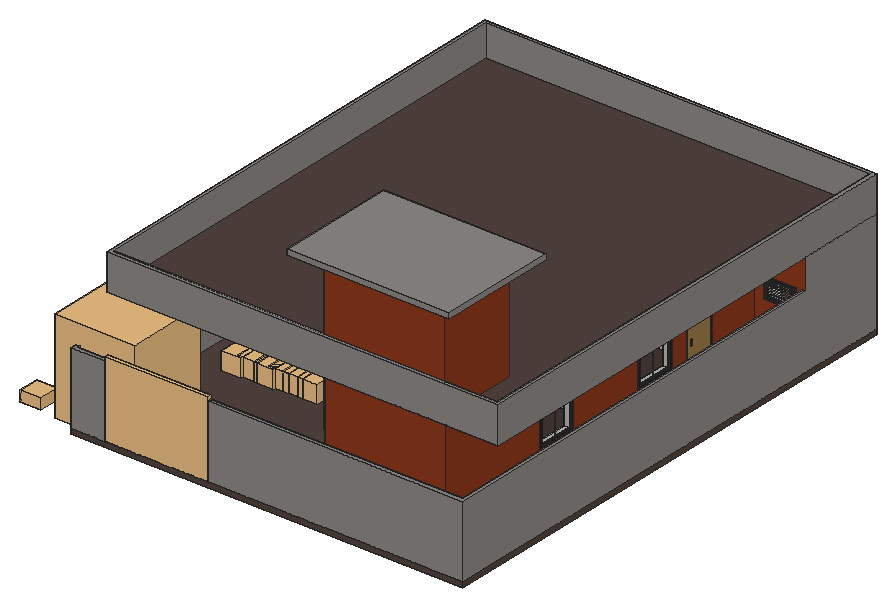
# SketchUp Ruby script. Lengths in inches.
U = 1.inch
M = Sketchup.active_model
def pt(a) = Geom::Point3d.new(a.map { |v| v * U })
def face(e, loops, mat)
  f = e.add_face(loops[0].map { |a| pt(a) })
  loops[1..].each { |l| e.add_face(l.map { |a| pt(a) }).erase! }
  f.material = f.back_material = mat if mat
  f
end
# faces: each face lists its corners as indices into pts; further lists are holes
def faces(e, pts, list, mat = nil) = list.each { |f| face(e, (f[0].is_a?(Array) ? f : [f]).map { |l| l.map { |i| pts[i] } }, mat) }
# xy, xz, yz: faces in a plane at the given z, y or x. An outline is a flat list of corners, or four numbers for a rectangle; further outlines are holes
def ring(l) = l.size == 4 ? [[l[0], l[1]], [l[2], l[1]], [l[2], l[3]], [l[0], l[3]]] : l.each_slice(2).to_a
def flat(e, list, mat, &to3) = list.each { |f| face(e, (f[0].is_a?(Array) ? f : [f]).map { |l| ring(l).map { |u, v| to3.(u, v) } }, mat) }
def xy(e, z, list, mat = nil) = flat(e, list, mat) { |x, y| [x, y, z] }
def xz(e, y, list, mat = nil) = flat(e, list, mat) { |x, z| [x, y, z] }
def yz(e, x, list, mat = nil) = flat(e, list, mat) { |y, z| [x, y, z] }
def lines(e, pts, list) = list.each { |a, b| e.add_line(pt(pts[a]), pt(pts[b])) }
# prism: a flat outline (further loops are holes) pulled along v
def prism(e, loops, v, mat = nil)
  f = face(e, loops, mat); d = Geom::Vector3d.new(v.map { |x| x * U })
  f.pushpull(f.normal.samedirection?(d) ? d.length : -d.length)
end
def box(e, o, s, mat = nil) = prism(e, [[o, [o[0] + s[0], o[1], o[2]], [o[0] + s[0], o[1] + s[1], o[2]], [o[0], o[1] + s[1], o[2]]]], [0, 0, s[2]], mat)
def at(x, y, z, deg = 0) = Geom::Transformation.translation(pt([x, y, z])) * Geom::Transformation.rotation(ORIGIN, Z_AXIS, deg.degrees)
def axes(o, x, y, z) = Geom::Transformation.new([*x, 0, *y, 0, *z, 0, *pt(o).to_a, 1])
def part(name) = M.definitions.add(name)
# library, detail: a bought-in or finely detailed component or shape, given as its bounding box
def library(name, o, s) = part(name).tap { |d| box(d.entities, o, s) }
def detail(e, o, s) = box(e.add_group.entities, o, s)
def put(e, d, t, mat = nil) = e.add_instance(d, t).tap { |i| i.material = mat if mat }
def group(e, t, mat = nil) = e.add_group.tap { |g| g.transformation = t; g.material = mat if mat }.entities
root = M.entities
M.materials.add("Aluminium Black Anodized 15cm").color = [38, 38, 38]
M.materials.add("Glass Yellow 001").color = [0, 0, 0]
M.materials["Glass Yellow 001"].alpha = 0.1
M.materials.add("Marble Emperador Dark 150cm").color = [81, 67, 62]
M.materials.add("Oak Northland Highgloss 300cm").color = [154, 122, 73]
M.materials.add("Wall Paint Autumn Maple Semigloss 300cm").color = [140, 56, 28]
M.materials.add("Wall Paint Poised Taupe Semigloss 300cm").color = [140, 135, 132]
c1 = library("Schefflera arboricola 003",[-47.85,-46.83,-0.79],[92.88,94.95,107.86])
c2 = library("Scabiosa atropurpurea 005",[-19.05,-18.08,-0.55],[34.7,36.31,33.14])
c3 = library("Skimmia japonica Rubella 004",[-17.08,-16.64,-0.26],[33.2,34.59,28.81])
c4 = library("Rubus caesius 001",[-11.39,-9.74,-0.56],[22.57,21.08,20.79])
c5 = library("gate 119k",[0,1.18,0],[135.43,4.73,99.21])
c6 = library("Dome Light",[-12,-12,0],[24,24,12])
c7 = part("Group\#13")
box(c7.entities,[0,0,0],[22,0.31,44])
put(root,c1,at(23.23,53.9,49.44))
put(root,c2,at(436.03,22.89,49.44))
put(root,c2,at(411.11,21.42,49.44))
put(root,c2,at(381.52,21.16,49.44))
put(root,c2,at(354.28,21.18,49.44))
put(root,c3,at(320.58,23.34,49.44))
put(root,c3,at(290.48,22.48,49.44))
put(root,c3,at(262.25,20.54,49.44))
put(root,c3,at(233.84,23.04,49.44))
put(root,c3,at(207.63,23.73,49.44))
put(root,c4,at(50.52,178.89,49.44))
put(root,c4,at(67.82,181.71,49.44))
put(root,c4,at(86.94,180.95,49.44))
put(root,c4,at(102.46,183.6,49.44))
put(root,c4,at(118.31,184.64,49.44))
put(root,c4,at(135.05,184.375,49.44))
put(root,c5,axes([39.15,-1.18,49.44],[0.88605,0,0],[0,1,0],[0,0,0.89]))
put(root,c6,at(-37.11,0,65.32))
g1 = group(root,at(0,0,49.44))
xy(g1,0,[[254.5,50.5,395.5,50.5,395.5,400.5,386.5,400.5,386.5,311.5,266.5,311.5,266.5,307,386.5,307,386.5,151,179.5,151,179.5,143,386.5,143,386.5,59.5,254.5,59.5],[391,507,447,507,447,591,391,591,391,579,386.5,579,386.5,543,391,543]])
xy(g1,36,[[240.1875,143,288.1875,151],[386.5,185.625,395.5,233.625],[75.8125,194,123.8125,203],[37,241.57,46,289.57],[386.5,328.1,395.5,376.1],
  [37,504.66,46,550.6875]])
xy(g1,60,[[37,337.54,46,373.54],[37,403.64,46,439.64],[408.25,498,444.25,507]])
xy(g1,84,[[240.1875,143,288.1875,151],[179.5,151,188.5,187],[386.5,185.625,395.5,233.625],[75.8125,194,123.8125,203],[37,241.57,46,289.57],
  [184,271.5,188.5,307.5],[82,319.5,118,324],[386.5,328.1,395.5,376.1],[37,337.54,46,373.54],[386.5,400.5,395.5,436.5],
  [37,403.64,46,439.64],[82,448.5,118,453],[166,448.5,202,453],[230.5,448.5,266.5,453],[408.25,498,444.25,507],
  [37,504.66,46,550.6875],[386.5,543,391,579]])
xy(g1,84,[[0,0,39.15,0,39.15,4.5,4.5,4.5,4.5,595.5,37,595.5,37,600,0,600],[159.15,0,456,0,456,498,451.5,498,451.5,4.5,159.15,4.5]],"Wall Paint Poised Taupe Semigloss 300cm")
xy(g1,120,[[[254.5,50.5,395.5,50.5,395.5,498,456,498,456,600,37,600,37,194,179.5,194,179.5,143,386.5,143,386.5,59.5,254.5,59.5],[188.5,151,188.5,324,134.5,324,134.5,448.5,386.5,448.5,386.5,311.5,266.5,311.5,266.5,307,386.5,307,386.5,151],[46,453,214,591],[218.5,453,386.5,591],[46,203,184,319.5],[46,324,130,384],[46,388.5,130,448.5],[391,507,447,591]]])
xz(g1,0,[[0,0,39.15,84],[159.15,0,456,84]],"Wall Paint Poised Taupe Semigloss 300cm")
xz(g1,4.5,[[4.5,0,39.15,84],[159.15,0,451.5,84]])
xz(g1,50.5,[[254.5,0,395.5,120]],"Wall Paint Autumn Maple Semigloss 300cm")
xz(g1,59.5,[[254.5,0,386.5,120]])
xz(g1,143,[[[179.5,0,386.5,120],[240.1875,36,288.1875,84]]],"Wall Paint Autumn Maple Semigloss 300cm")
xz(g1,151,[[[179.5,0,179.5,84,188.5,84,188.5,120,386.5,120,386.5,0],[240.1875,36,288.1875,84]]])
xz(g1,185.625,[[386.5,36,395.5,84]])
xz(g1,187,[[179.5,0,188.5,84]])
xz(g1,194,[[[37,0,179.5,120],[75.8125,36,123.8125,84]]],"Wall Paint Autumn Maple Semigloss 300cm")
xz(g1,203,[[[46,0,184,120],[75.8125,36,123.8125,84]]])
xz(g1,233.625,[[386.5,36,395.5,84]])
xz(g1,241.57,[[37,36,46,84]])
xz(g1,271.5,[[184,0,188.5,84]])
xz(g1,289.57,[[37,36,46,84]])
xz(g1,307,[[266.5,0,386.5,120]])
xz(g1,307.5,[[184,0,188.5,84]])
xz(g1,311.5,[[266.5,0,386.5,120]])
xz(g1,319.5,[[46,0,82,0,82,84,118,84,118,0,184,0,184,120,46,120]])
xz(g1,324,[[46,0,46,120,130,120,130,0,118,0,118,84,82,84,82,0],[134.5,0,188.5,120]])
xz(g1,328.1,[[386.5,36,395.5,84]])
xz(g1,337.54,[[37,60,46,84]])
xz(g1,373.54,[[37,60,46,84]])
xz(g1,376.1,[[386.5,36,395.5,84]])
xz(g1,384,[[46,0,130,120]])
xz(g1,388.5,[[46,0,130,120]])
xz(g1,400.5,[[386.5,0,395.5,84]])
xz(g1,403.64,[[37,60,46,84]])
xz(g1,436.5,[[386.5,0,395.5,84]])
xz(g1,439.64,[[37,60,46,84]])
xz(g1,448.5,[[46,0,82,0,82,84,118,84,118,0,130,0,130,120,46,120],[134.5,0,166,0,166,84,202,84,202,0,230.5,0,230.5,84,266.5,84,266.5,0,386.5,0,386.5,120,134.5,120]])
xz(g1,453,[[46,0,46,120,214,120,214,0,202,0,202,84,166,84,166,0,118,0,118,84,82,84,82,0],[218.5,0,218.5,120,386.5,120,386.5,0,266.5,0,266.5,84,230.5,84,230.5,0]])
xz(g1,498,[[[395.5,0,451.5,0,451.5,84,456,84,456,120,395.5,120],[408.25,60,444.25,84]]],"Wall Paint Autumn Maple Semigloss 300cm")
xz(g1,504.66,[[37,36,46,84]])
xz(g1,507,[[[391,0,447,120],[408.25,60,444.25,84]]])
xz(g1,543,[[386.5,0,391,84]])
xz(g1,550.6875,[[37,36,46,84]])
xz(g1,579,[[386.5,0,391,84]])
xz(g1,591,[[46,0,214,120],[218.5,0,386.5,120],[391,0,447,120]])
xz(g1,595.5,[[4.5,0,37,84]],"Wall Paint Poised Taupe Semigloss 300cm")
xz(g1,600,[[0,0,0,84,37,84,37,120,456,120,456,0]],"Wall Paint Poised Taupe Semigloss 300cm")
yz(g1,0,[[0,0,600,84]],"Wall Paint Poised Taupe Semigloss 300cm")
yz(g1,4.5,[[4.5,0,595.5,84]],"Wall Paint Poised Taupe Semigloss 300cm")
yz(g1,37,[[[194,0,194,120,600,120,600,84,595.5,84,595.5,0],[241.57,36,289.57,84],[504.66,36,550.6875,84],[403.64,60,439.64,84],[337.54,60,373.54,84]]],"Wall Paint Autumn Maple Semigloss 300cm")
yz(g1,39.15,[[0,0,4.5,84]],"Wall Paint Poised Taupe Semigloss 300cm")
yz(g1,46,[[[203,0,319.5,120],[241.57,36,289.57,84]],[[324,0,384,120],[337.54,60,373.54,84]],[[388.5,0,448.5,120],[403.64,60,439.64,84]],[[453,0,591,120],[504.66,36,550.6875,84]]])
yz(g1,75.8125,[[194,36,203,84]])
yz(g1,82,[[319.5,0,324,84],[448.5,0,453,84]])
yz(g1,118,[[319.5,0,324,84],[448.5,0,453,84]])
yz(g1,123.8125,[[194,36,203,84]])
yz(g1,130,[[324,0,384,120],[388.5,0,448.5,120]])
yz(g1,134.5,[[324,0,448.5,120]])
yz(g1,159.15,[[0,0,4.5,84]],"Wall Paint Poised Taupe Semigloss 300cm")
yz(g1,166,[[448.5,0,453,84]])
yz(g1,179.5,[[143,0,143,120,194,120,194,0,187,0,187,84,151,84,151,0]],"Wall Paint Autumn Maple Semigloss 300cm")
yz(g1,184,[[203,0,203,120,319.5,120,319.5,0,307.5,0,307.5,84,271.5,84,271.5,0]])
yz(g1,188.5,[[187,0,271.5,0,271.5,84,307.5,84,307.5,0,324,0,324,120,151,120,151,84,187,84]])
yz(g1,202,[[448.5,0,453,84]])
yz(g1,214,[[453,0,591,120]])
yz(g1,218.5,[[453,0,591,120]])
yz(g1,230.5,[[448.5,0,453,84]])
yz(g1,240.1875,[[143,36,151,84]])
yz(g1,254.5,[[50.5,0,59.5,120]])
yz(g1,266.5,[[307,0,311.5,120],[448.5,0,453,84]])
yz(g1,288.1875,[[143,36,151,84]])
yz(g1,386.5,[[59.5,0,143,120],[[151,0,307,120],[185.625,36,233.625,84]],[[311.5,0,311.5,120,448.5,120,448.5,0,436.5,0,436.5,84,400.5,84,400.5,0],[328.1,36,376.1,84]],[453,0,453,120,591,120,591,0,579,0,579,84,543,84,543,0]])
yz(g1,391,[[507,0,543,0,543,84,579,84,579,0,591,0,591,120,507,120]])
yz(g1,395.5,[[[50.5,0,400.5,0,400.5,84,436.5,84,436.5,0,498,0,498,120,50.5,120],[328.1,36,376.1,84],[185.625,36,233.625,84]]],"Wall Paint Autumn Maple Semigloss 300cm")
yz(g1,408.25,[[498,60,507,84]])
yz(g1,444.25,[[498,60,507,84]])
yz(g1,447,[[507,0,591,120]])
yz(g1,451.5,[[4.5,0,498,84]],"Wall Paint Poised Taupe Semigloss 300cm")
yz(g1,456,[[0,0,600,0,600,120,498,120,498,84,0,84]],"Wall Paint Poised Taupe Semigloss 300cm")
g2 = group(g1,at(254.5,101.25,0))
box(g2,[0,0,0],[12,41.75,7.06])
g3 = group(g1,at(266.5,101.25,7.06))
box(g3,[0,0,0],[12,41.75,7.06])
g4 = group(g1,at(278.5,101.25,14.12))
box(g4,[0,0,0],[12,41.75,7.06])
g5 = group(g1,at(290.5,101.25,21.18))
box(g5,[0,0,0],[12,41.75,7.06])
g6 = group(g1,at(302.5,101.25,28.24))
box(g6,[0,0,0],[12,41.75,7.06])
g7 = group(g1,at(314.5,101.25,35.3))
box(g7,[0,0,0],[12,41.75,7.06])
g8 = group(g1,at(326.5,101.25,42.36))
box(g8,[0,0,0],[12,41.75,7.06])
g9 = group(g1,at(338.5,101.25,49.42))
box(g9,[0,0,0],[12,41.75,7.06])
g10 = group(g1,at(350.5,101.25,56.48))
box(g10,[0,-41.75,0],[36,83.5,7.06])
g11 = group(g1,at(338.5,59.5,63.54))
box(g11,[0,0,0],[12,41.75,7.06])
g12 = group(g1,at(326.5,59.5,70.6))
box(g12,[0,0,0],[12,41.75,7.06])
g13 = group(g1,at(314.5,59.5,77.66))
box(g13,[0,0,0],[12,41.75,7.06])
g14 = group(g1,at(302.5,59.5,84.72))
box(g14,[0,0,0],[12,41.75,7.06])
g15 = group(g1,at(290.5,59.5,91.78))
box(g15,[0,0,0],[12,41.75,7.06])
g16 = group(g1,at(278.5,59.5,98.84))
box(g16,[0,0,0],[12,41.75,7.06])
g17 = group(g1,at(266.5,59.5,105.9))
box(g17,[0,0,0],[12,41.75,7.06])
g18 = group(g1,at(254.5,59.5,112.96))
box(g18,[0,0,0],[12,41.75,7.06])
g19 = group(g1,at(37,504.66,36))
prism(g19,[[[1.5,0,48],[1.5,0,0],[1.5,46.02,0],[1.5,46.02,48]],[[1.5,2,46],[1.5,44.02,46],[1.5,44.02,2],[1.5,2,2]]],[-3,0,0],"Aluminium Black Anodized 15cm")
g20 = group(g19,at(0.3125,23.01,2),"Glass Yellow 001")
box(g20,[0,0,0],[0.31,21.01,44],"Glass Yellow 001")
g21 = group(g19,at(0,2,2),"Glass Yellow 001")
box(g21,[0,0,0],[0.31,21.01,44],"Glass Yellow 001")
g22 = group(g1,at(37,403.64,60))
prism(g22,[[[-1.5,0,0],[-1.5,0,24],[-1.5,36,24],[-1.5,36,0]],[[-1.5,2,22],[-1.5,2,2],[-1.5,34,2],[-1.5,34,22]]],[3,0,0],"Aluminium Black Anodized 15cm")
g23 = group(g22,at(-1.5,2,20),"Glass Yellow 001")
box(g23,[0,0,0],[0.31,32,2],"Glass Yellow 001")
g24 = group(g22,at(-1.5,2,17),"Glass Yellow 001")
box(g24,[0,0,0],[0.31,32,2],"Glass Yellow 001")
g25 = group(g22,at(-1.5,2,14),"Glass Yellow 001")
box(g25,[0,0,0],[0.31,32,2],"Glass Yellow 001")
g26 = group(g22,at(-1.5,2,11),"Glass Yellow 001")
box(g26,[0,0,0],[0.31,32,2],"Glass Yellow 001")
g27 = group(g22,at(-1.5,2,8),"Glass Yellow 001")
box(g27,[0,0,0],[0.31,32,2],"Glass Yellow 001")
g28 = group(g22,at(-1.5,2,5),"Glass Yellow 001")
box(g28,[0,0,0],[0.31,32,2],"Glass Yellow 001")
g29 = group(g22,at(-1.5,2,2),"Glass Yellow 001")
box(g29,[0,0,0],[0.31,32,2],"Glass Yellow 001")
g30 = group(g1,at(37,337.54,60))
prism(g30,[[[-1.5,0,0],[-1.5,0,24],[-1.5,36,24],[-1.5,36,0]],[[-1.5,2,22],[-1.5,2,2],[-1.5,34,2],[-1.5,34,22]]],[3,0,0],"Aluminium Black Anodized 15cm")
g31 = group(g30,at(-1.5,2,20),"Glass Yellow 001")
box(g31,[0,0,0],[0.31,32,2],"Glass Yellow 001")
g32 = group(g30,at(-1.5,2,17),"Glass Yellow 001")
box(g32,[0,0,0],[0.31,32,2],"Glass Yellow 001")
g33 = group(g30,at(-1.5,2,14),"Glass Yellow 001")
box(g33,[0,0,0],[0.31,32,2],"Glass Yellow 001")
g34 = group(g30,at(-1.5,2,11),"Glass Yellow 001")
box(g34,[0,0,0],[0.31,32,2],"Glass Yellow 001")
g35 = group(g30,at(-1.5,2,8),"Glass Yellow 001")
box(g35,[0,0,0],[0.31,32,2],"Glass Yellow 001")
g36 = group(g30,at(-1.5,2,5),"Glass Yellow 001")
box(g36,[0,0,0],[0.31,32,2],"Glass Yellow 001")
g37 = group(g30,at(-1.5,2,2),"Glass Yellow 001")
box(g37,[0,0,0],[0.31,32,2],"Glass Yellow 001")
g38 = group(g1,at(37,241.57,36))
prism(g38,[[[-1.5,0,0],[-1.5,0,48],[-1.5,48,48],[-1.5,48,0]],[[-1.5,2,46],[-1.5,2,2],[-1.5,46,2],[-1.5,46,46]]],[3,0,0],"Aluminium Black Anodized 15cm")
g39 = group(g38,at(-0.0625,24,2),"Glass Yellow 001")
box(g39,[0,0,0],[0.31,22,44],"Glass Yellow 001")
g40 = group(g38,at(-0.38,2,2),"Glass Yellow 001")
box(g40,[0,0,0],[0.31,22,44],"Glass Yellow 001")
g41 = group(g1,at(75.8125,194,36))
prism(g41,[[[0,-1.5,0],[48,-1.5,0],[48,-1.5,48],[0,-1.5,48]],[[46,-1.5,46],[46,-1.5,2],[2,-1.5,2],[2,-1.5,46]]],[0,3,0],"Aluminium Black Anodized 15cm")
g42 = group(g41,at(2,0.4375,2),"Glass Yellow 001")
box(g42,[0,0,0],[22,0.31,44],"Glass Yellow 001")
g43 = group(g41,at(24,0.12,1.64),"Glass Yellow 001")
box(g43,[0,0,0],[22,0.31,44],"Glass Yellow 001")
g44 = group(g1,at(395.5,185.625,36))
prism(g44,[[[1.5,0,0],[1.5,48,0],[1.5,48,48],[1.5,0,48]],[[1.5,46,46],[1.5,46,2],[1.5,2,2],[1.5,2,46]]],[-3,0,0],"Aluminium Black Anodized 15cm")
g45 = group(g44,at(-0.25,2,2),"Glass Yellow 001")
box(g45,[-0.31,0,0],[0.31,22,44],"Glass Yellow 001")
g46 = group(g44,at(0.06,24,2),"Glass Yellow 001")
box(g46,[-0.31,0,0],[0.31,22,44],"Glass Yellow 001")
g47 = group(g1,at(395.5,328.1,36))
prism(g47,[[[1.5,48,0],[1.5,48,48],[1.5,0,48],[1.5,0,0]],[[1.5,46,46],[1.5,46,2],[1.5,2,2],[1.5,2,46]]],[-3,0,0],"Aluminium Black Anodized 15cm")
g48 = group(g47,at(-0.5,2,2),"Glass Yellow 001")
box(g48,[-0.31,0,0],[0.31,22,44],"Glass Yellow 001")
g49 = group(g47,at(-0.19,24,2),"Glass Yellow 001")
box(g49,[-0.31,0,0],[0.31,22,44],"Glass Yellow 001")
g50 = group(g1,at(408.25,498,60))
prism(g50,[[[0,-1.5,0],[36,-1.5,0],[36,-1.5,24],[0,-1.5,24]],[[34,-1.5,22],[34,-1.5,2],[2,-1.5,2],[2,-1.5,22]]],[0,3,0],"Aluminium Black Anodized 15cm")
g51 = group(g50,at(2,-1.5,20),"Glass Yellow 001")
box(g51,[0,-0.31,0],[32,0.31,2],"Glass Yellow 001")
g52 = group(g50,at(2,-1.5,17),"Glass Yellow 001")
box(g52,[0,-0.31,0],[32,0.31,2],"Glass Yellow 001")
g53 = group(g50,at(2,-1.5,14),"Glass Yellow 001")
box(g53,[0,-0.31,0],[32,0.31,2],"Glass Yellow 001")
g54 = group(g50,at(2,-1.5,11),"Glass Yellow 001")
box(g54,[0,-0.31,0],[32,0.31,2],"Glass Yellow 001")
g55 = group(g50,at(2,-1.5,8),"Glass Yellow 001")
box(g55,[0,-0.31,0],[32,0.31,2],"Glass Yellow 001")
g56 = group(g50,at(2,-1.5,5),"Glass Yellow 001")
box(g56,[0,-0.31,0],[32,0.31,2],"Glass Yellow 001")
g57 = group(g50,at(2,-1.5,2),"Glass Yellow 001")
box(g57,[0,-0.31,0],[32,0.31,2],"Glass Yellow 001")
g58 = group(g1,at(179.5,151,0))
xy(g58,0,[[0,0,2.5,36]])
xy(g58,2,[[0,2,2.5,34]])
xy(g58,82,[[0,2,2.5,34]])
xy(g58,84,[[0,0,2.5,36]])
xz(g58,0,[[0,0,2.5,84]])
xz(g58,2,[[0,2,2.5,82]])
xz(g58,34,[[0,2,2.5,82]])
xz(g58,36,[[0,0,2.5,84]])
yz(g58,0,[[[0,0,36,84],[2,2,34,82]]],"Aluminium Black Anodized 15cm")
yz(g58,2.5,[[[0,0,36,84],[2,2,34,82]]])
g59 = group(g58,at(0,2,2),"Oak Northland Highgloss 300cm")
box(g59,[0,0,0],[0.71,32,80],"Oak Northland Highgloss 300cm")
g60 = group(g58,at(0,27.21,35.97),"Aluminium Black Anodized 15cm")
box(g60,[-0.5,0,0],[0.5,1.99,6.86],"Aluminium Black Anodized 15cm")
g61 = group(g1,at(188.5,271.5,0))
prism(g61,[[[0,36,0],[0,36,84],[0,0,84],[0,0,0]],[[0,2,82],[0,34,82],[0,34,2],[0,2,2]]],[-2.5,0,0],"Aluminium Black Anodized 15cm")
g62 = group(g61,at(0,2,2))
box(g62,[-0.71,0,0],[0.71,32,80],"Oak Northland Highgloss 300cm")
g63 = group(g61,at(0,4.64,43.75))
box(g63,[0,0,0],[0.5,1.75,7.1875],"Aluminium Black Anodized 15cm")
g64 = group(g1,at(82,319.5,0))
prism(g64,[[[36,0,0],[36,0,84],[0,0,84],[0,0,0]],[[2,0,82],[34,0,82],[34,0,2],[2,0,2]]],[0,2.5,0],"Aluminium Black Anodized 15cm")
g65 = group(g64,at(2,0,2),"Oak Northland Highgloss 300cm")
box(g65,[0,0,0],[32,0.71,80],"Oak Northland Highgloss 300cm")
g66 = group(g65,at(3.92,0,37.52),"Aluminium Black Anodized 15cm")
xy(g66,0,[[0,-0.5,1.375,0]])
xy(g66,6.0625,[[0,-0.5,1.375,0]])
xz(g66,-0.5,[[0,0,1.375,6.0625]])
xz(g66,0,[[0,0,1.375,6.0625]])
yz(g66,0,[[-0.5,0,0,6.0625]],"Aluminium Black Anodized 15cm")
yz(g66,1.375,[[-0.5,0,0,6.0625]],"Aluminium Black Anodized 15cm")
g67 = group(g1,at(166,448.5,0))
prism(g67,[[[0,0,0],[36,0,0],[36,0,84],[0,0,84]],[[2,0,82],[34,0,82],[34,0,2],[2,0,2]]],[0,2.5,0],"Aluminium Black Anodized 15cm")
g68 = group(g67,at(2,0,2))
box(g68,[0,0,0],[32,0.71,80],"Oak Northland Highgloss 300cm")
g69 = group(g68,at(3,0,41.125),"Aluminium Black Anodized 15cm")
box(g69,[0,-0.5,0],[1.5,0.5,6.0625],"Aluminium Black Anodized 15cm")
g70 = group(g1,at(230.5,448.5,0))
prism(g70,[[[36,0,0],[36,0,84],[0,0,84],[0,0,0]],[[34,0,82],[34,0,2],[2,0,2],[2,0,82]]],[0,2.5,0],"Aluminium Black Anodized 15cm")
g71 = group(g70,at(2,0,2))
box(g71,[0,0,0],[32,0.71,80],"Oak Northland Highgloss 300cm")
g72 = group(g71,at(4.01,0,40.92),"Aluminium Black Anodized 15cm")
box(g72,[0,-0.5,0],[1.3125,0.5,5],"Aluminium Black Anodized 15cm")
g73 = group(g1,at(386.5,543,0))
xy(g73,0,[[0,0,2.5,36]])
xy(g73,2,[[0,2,2.5,34]])
xy(g73,82,[[0,2,2.5,34]])
xy(g73,84,[[0,0,2.5,36]])
xz(g73,0,[[0,0,2.5,84]])
xz(g73,2,[[0,2,2.5,82]])
xz(g73,34,[[0,2,2.5,82]])
xz(g73,36,[[0,0,2.5,84]])
yz(g73,0,[[[0,0,36,84],[2,2,34,82]]],"Aluminium Black Anodized 15cm")
yz(g73,2.5,[[[0,0,36,84],[2,2,34,82]]])
g74 = group(g73,at(0,2,2))
box(g74,[0,0,0],[0.71,32,80],"Oak Northland Highgloss 300cm")
g75 = group(g74,at(0,28.83,39.84),"Aluminium Black Anodized 15cm")
box(g75,[-0.5,-1.8125,0],[0.5,1.8125,7.1875],"Aluminium Black Anodized 15cm")
g76 = group(g74,at(-304.5,-92,-2))
xy(g76,0,[[0,-2.5,36,0]])
xy(g76,2,[[2,-2.5,34,0]])
xy(g76,82,[[2,-2.5,34,0]])
xy(g76,84,[[0,-2.5,36,0]])
xz(g76,-2.5,[[[0,0,36,84],[2,2,34,82]]])
xz(g76,0,[[[0,0,36,84],[2,2,34,82]]],"Aluminium Black Anodized 15cm")
yz(g76,0,[[-2.5,0,0,84]])
yz(g76,2,[[-2.5,2,0,82]])
yz(g76,34,[[-2.5,2,0,82]])
yz(g76,36,[[-2.5,0,0,84]])
g77 = group(g76,at(2,0,2))
box(g77,[0,-0.71,0],[32,0.71,80],"Oak Northland Highgloss 300cm")
g78 = group(g77,at(27.99,0,35.91),"Aluminium Black Anodized 15cm")
box(g78,[-1.125,0,0],[1.125,0.5,6.9375],"Aluminium Black Anodized 15cm")
g79 = group(g1,at(395.5,400.5,0))
prism(g79,[[[0,36,0],[0,36,84],[0,0,84],[0,0,0]],[[0,2,2],[0,2,82],[0,34,82],[0,34,2]]],[-2.5,0,0],"Aluminium Black Anodized 15cm")
g80 = group(g79,at(0,2,2),"Oak Northland Highgloss 300cm")
box(g80,[-0.71,0,0],[0.71,32,80],"Oak Northland Highgloss 300cm")
g81 = group(g79,at(0,5.25,46.25),"Aluminium Black Anodized 15cm")
box(g81,[0,0,0],[0.5,1.5,7.0625],"Aluminium Black Anodized 15cm")
g82 = group(root,at(240.1875,143,85.44))
prism(g82,[[[48,-1.5,0],[48,-1.5,48],[0,-1.5,48],[0,-1.5,0]],[[2,-1.5,2],[2,-1.5,46],[46,-1.5,46],[46,-1.5,2]]],[0,3,0],"Aluminium Black Anodized 15cm")
put(g82,c7,at(2,0,2),"Glass Yellow 001")
put(g82,c7,at(24,-0.31,2),"Glass Yellow 001")
g83 = group(root,at(37,50.5,169.44))
xy(g83,0,[[[-36,0,419,549.5],[217.5,9,349.25,92.5]]])
xy(g83,6,[[-31.5,4.5,213,4.5,213,9,217.5,9,217.5,50.75,213,50.75,213,97,353.75,97,353.75,4.5,414.5,4.5,414.5,545,-31.5,545]],"Marble Emperador Dark 150cm")
xy(g83,42,[[[-36,0,419,549.5],[-31.5,4.5,414.5,545]]],"Wall Paint Poised Taupe Semigloss 300cm")
xy(g83,90,[[213,9,217.5,50.75]])
xy(g83,126,[[[213,4.5,353.75,97],[217.5,9,349.25,92.5]]])
xz(g83,0,[[-36,0,419,42]],"Wall Paint Poised Taupe Semigloss 300cm")
xz(g83,4.5,[[213,42,353.75,126]],"Wall Paint Autumn Maple Semigloss 300cm")
xz(g83,4.5,[[-31.5,6,213,42],[353.75,6,414.5,42]],"Wall Paint Poised Taupe Semigloss 300cm")
xz(g83,9,[[217.5,0,217.5,6,213,6,213,90,217.5,90,217.5,126,349.25,126,349.25,0]])
xz(g83,50.75,[[213,6,217.5,90]])
xz(g83,92.5,[[217.5,0,349.25,126]])
xz(g83,97,[[213,6,353.75,126]],"Wall Paint Autumn Maple Semigloss 300cm")
xz(g83,545,[[-31.5,6,414.5,42]],"Wall Paint Poised Taupe Semigloss 300cm")
xz(g83,549.5,[[-36,0,419,42]],"Wall Paint Poised Taupe Semigloss 300cm")
yz(g83,-36,[[0,0,549.5,42]],"Wall Paint Poised Taupe Semigloss 300cm")
yz(g83,-31.5,[[4.5,6,545,42]],"Wall Paint Poised Taupe Semigloss 300cm")
yz(g83,213,[[4.5,6,4.5,126,97,126,97,6,50.75,6,50.75,90,9,90,9,6]],"Wall Paint Autumn Maple Semigloss 300cm")
yz(g83,217.5,[[9,0,92.5,0,92.5,126,9,126,9,90,50.75,90,50.75,6,9,6]])
yz(g83,349.25,[[9,0,92.5,126]])
yz(g83,353.75,[[4.5,6,97,126]],"Wall Paint Autumn Maple Semigloss 300cm")
yz(g83,414.5,[[4.5,6,545,42]],"Wall Paint Poised Taupe Semigloss 300cm")
yz(g83,419,[[0,0,549.5,42]],"Wall Paint Poised Taupe Semigloss 300cm")
g84 = group(g83,at(213,9,6))
xy(g84,0,[[0,0,2,41.75]])
xy(g84,2,[[0,2,2,39.75]])
xy(g84,82,[[0,2,2,39.75]])
xy(g84,84,[[0,0,2,41.75]])
xz(g84,0,[[0,0,2,84]])
xz(g84,2,[[0,2,2,82]])
xz(g84,39.75,[[0,2,2,82]])
xz(g84,41.75,[[0,0,2,84]])
yz(g84,0,[[[0,0,41.75,84],[2,2,39.75,82]]],"Aluminium Black Anodized 15cm")
yz(g84,2,[[[0,0,41.75,84],[2,2,39.75,82]]])
g85 = group(g84,at(0,2,2))
xy(g85,0,[[0,0,0.71,37.75]])
xy(g85,80,[[0,0,0.71,37.75]])
xz(g85,0,[[0,0,0.71,80]])
xz(g85,37.75,[[0,0,0.71,80]])
yz(g85,0,[[0,0,37.75,80]],"Oak Northland Highgloss 300cm")
yz(g85,0.71,[[0,0,37.75,80]])
g86 = group(g85,at(0,34.59,42.55),"Aluminium Black Anodized 15cm")
box(g86,[-0.5,-1.5625,0],[0.5,1.5625,6.6875],"Aluminium Black Anodized 15cm")
g87 = group(root,at(250,55,295.44),"Wall Paint Poised Taupe Semigloss 300cm")
box(g87,[-24,-24,0],[188.75,140.5,6],"Wall Paint Poised Taupe Semigloss 300cm")
g88 = group(root,at(0,0,49.44),"Marble Emperador Dark 150cm")
box(g88,[0,0,-6],[456,600,6],"Marble Emperador Dark 150cm")
